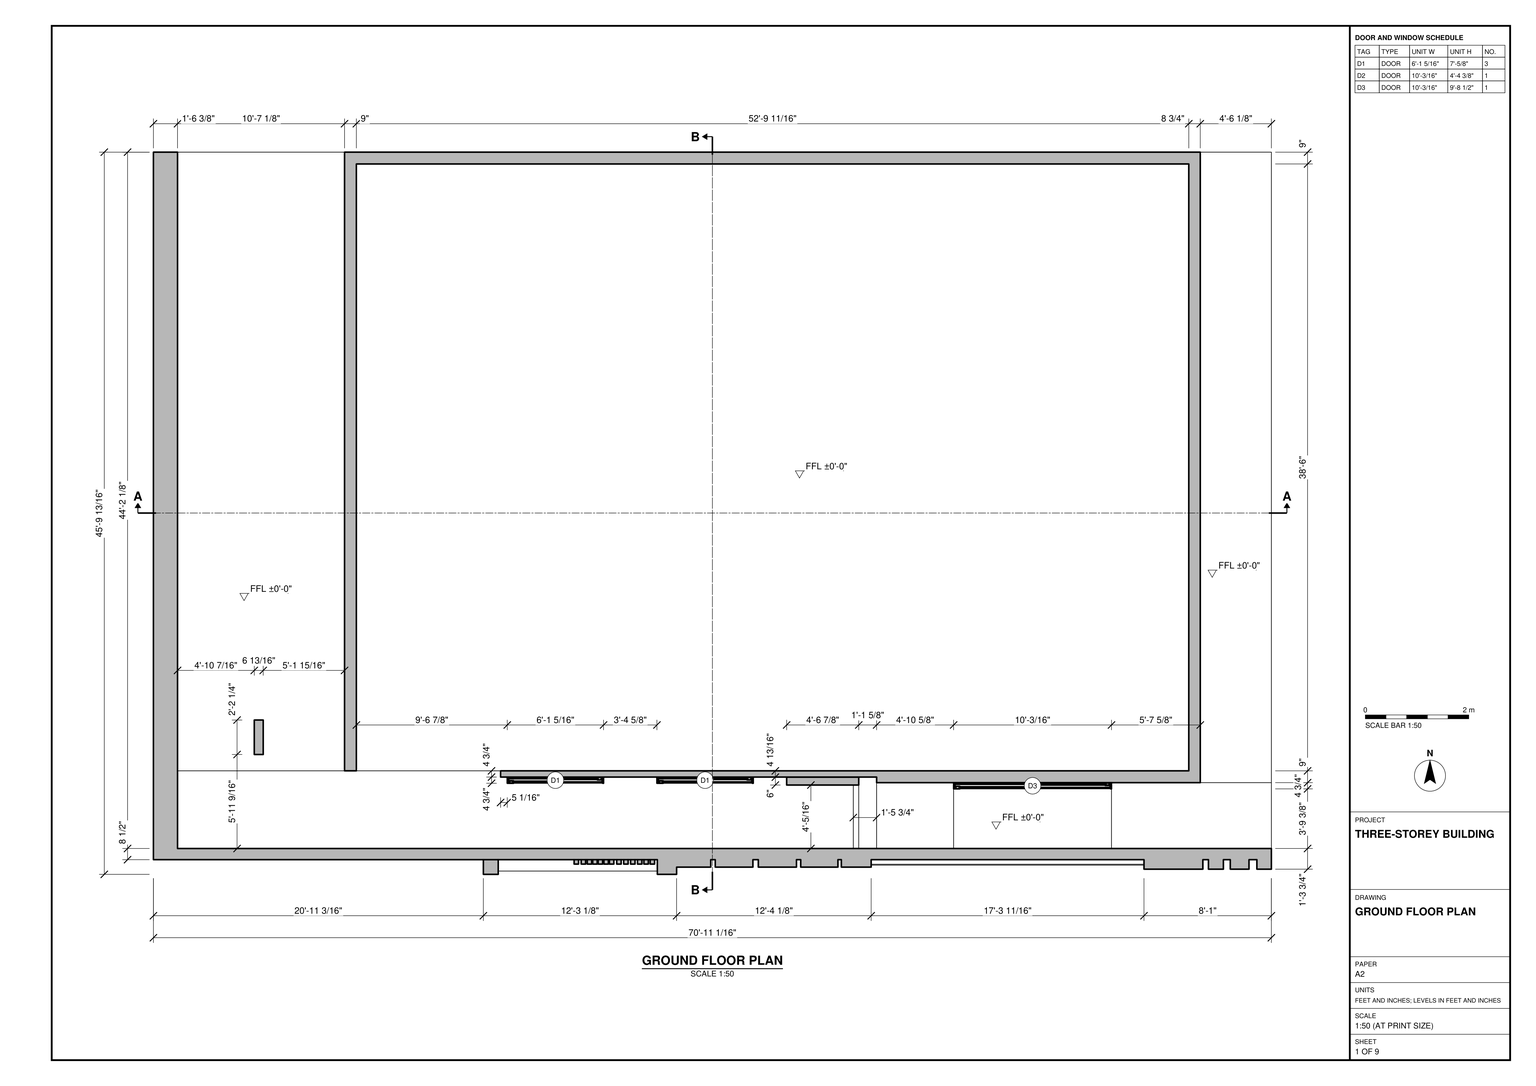
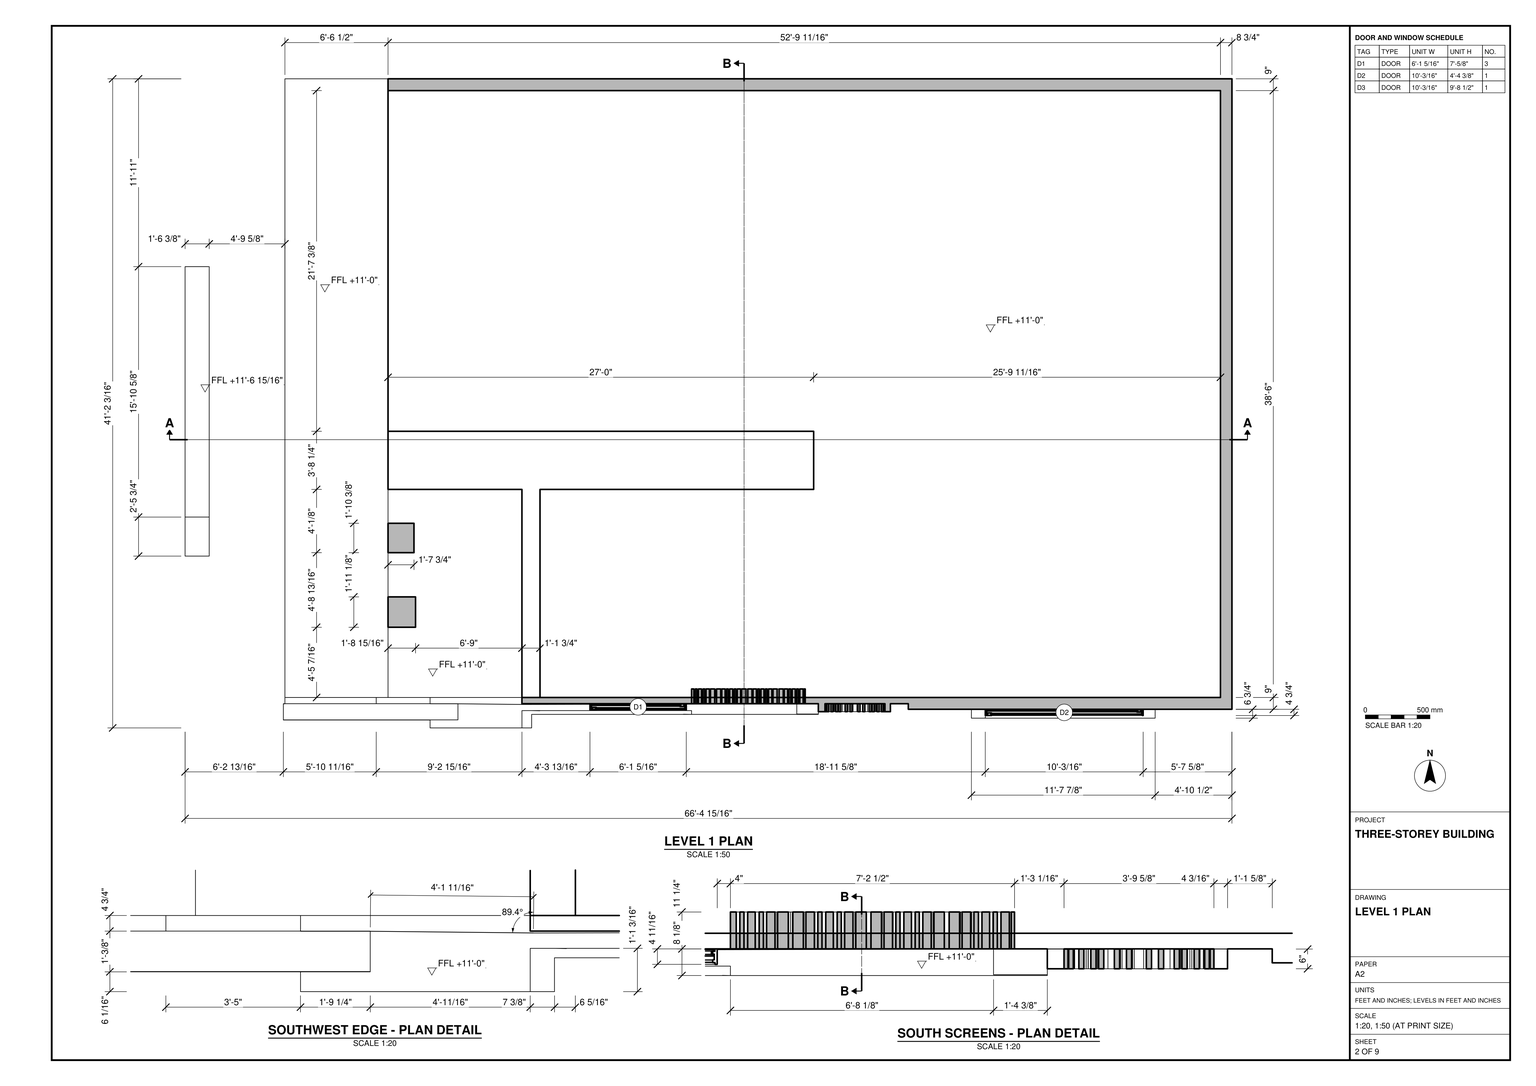
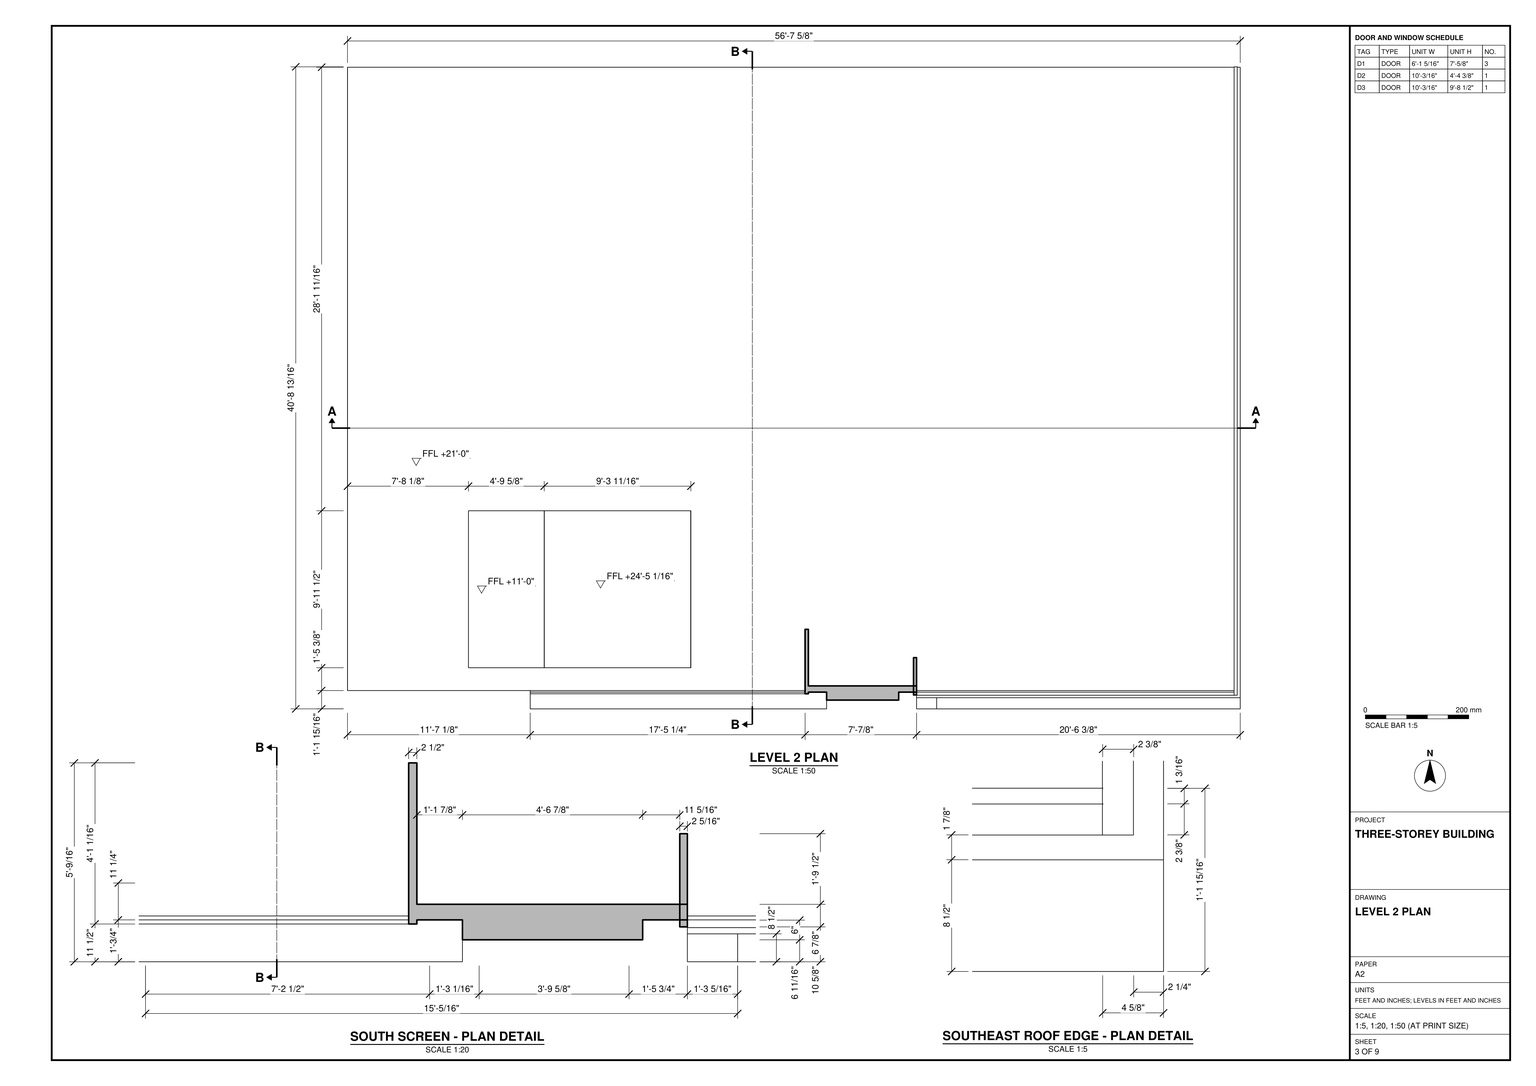
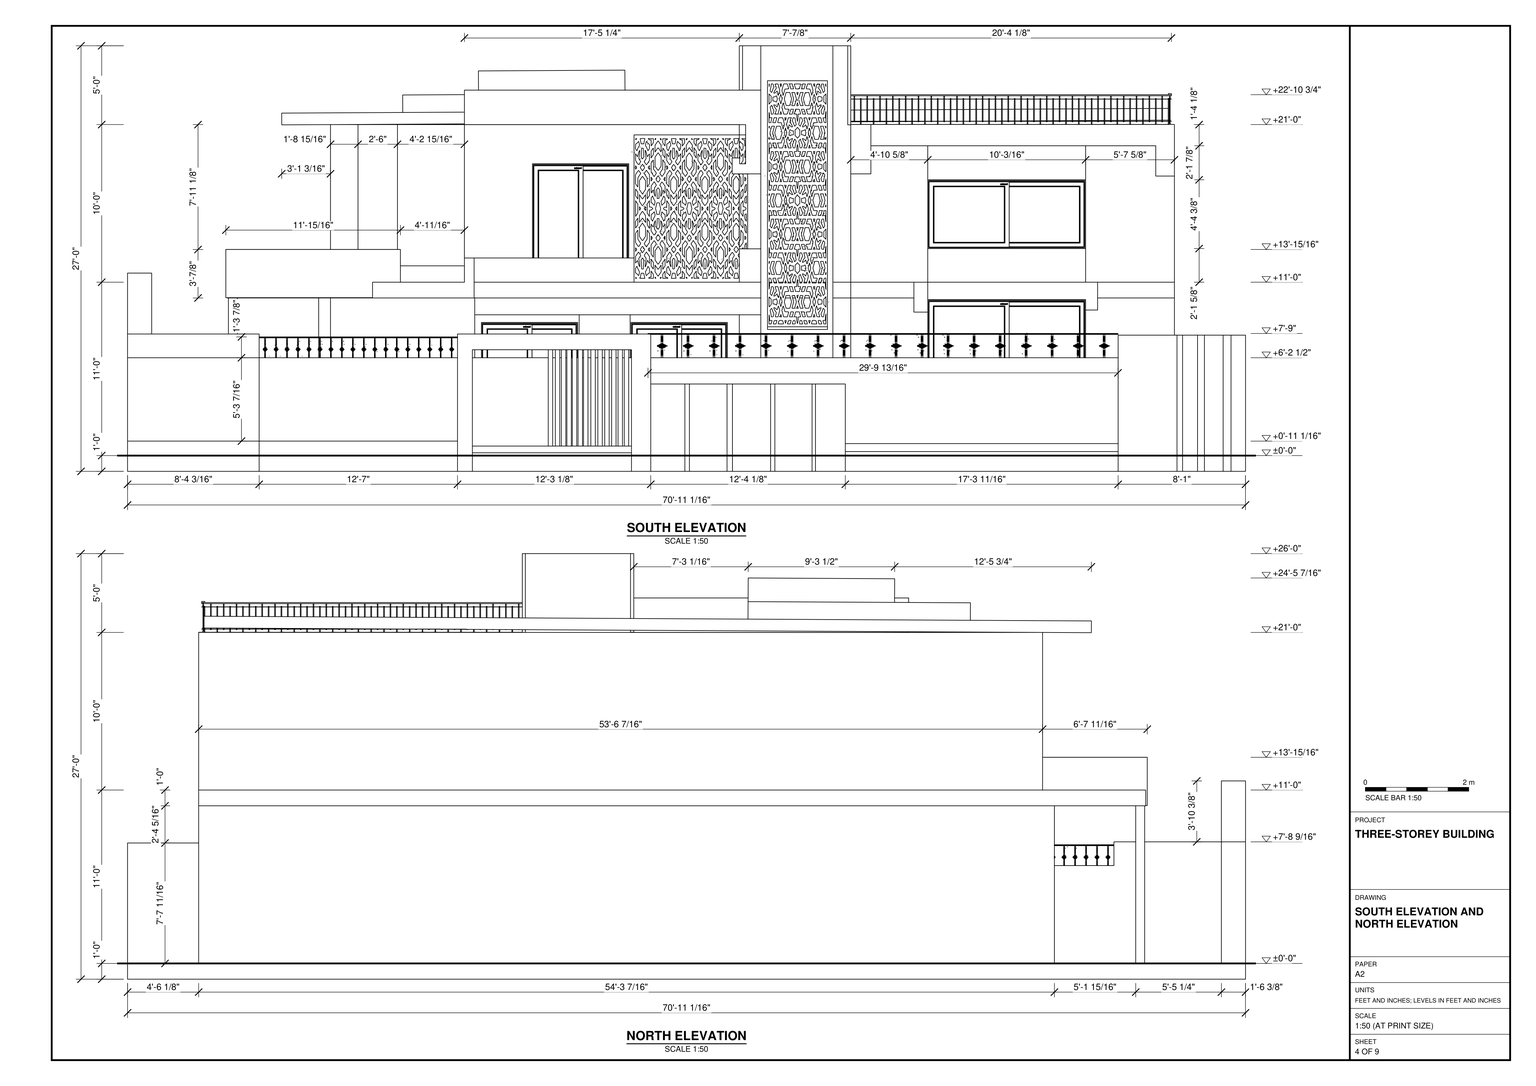
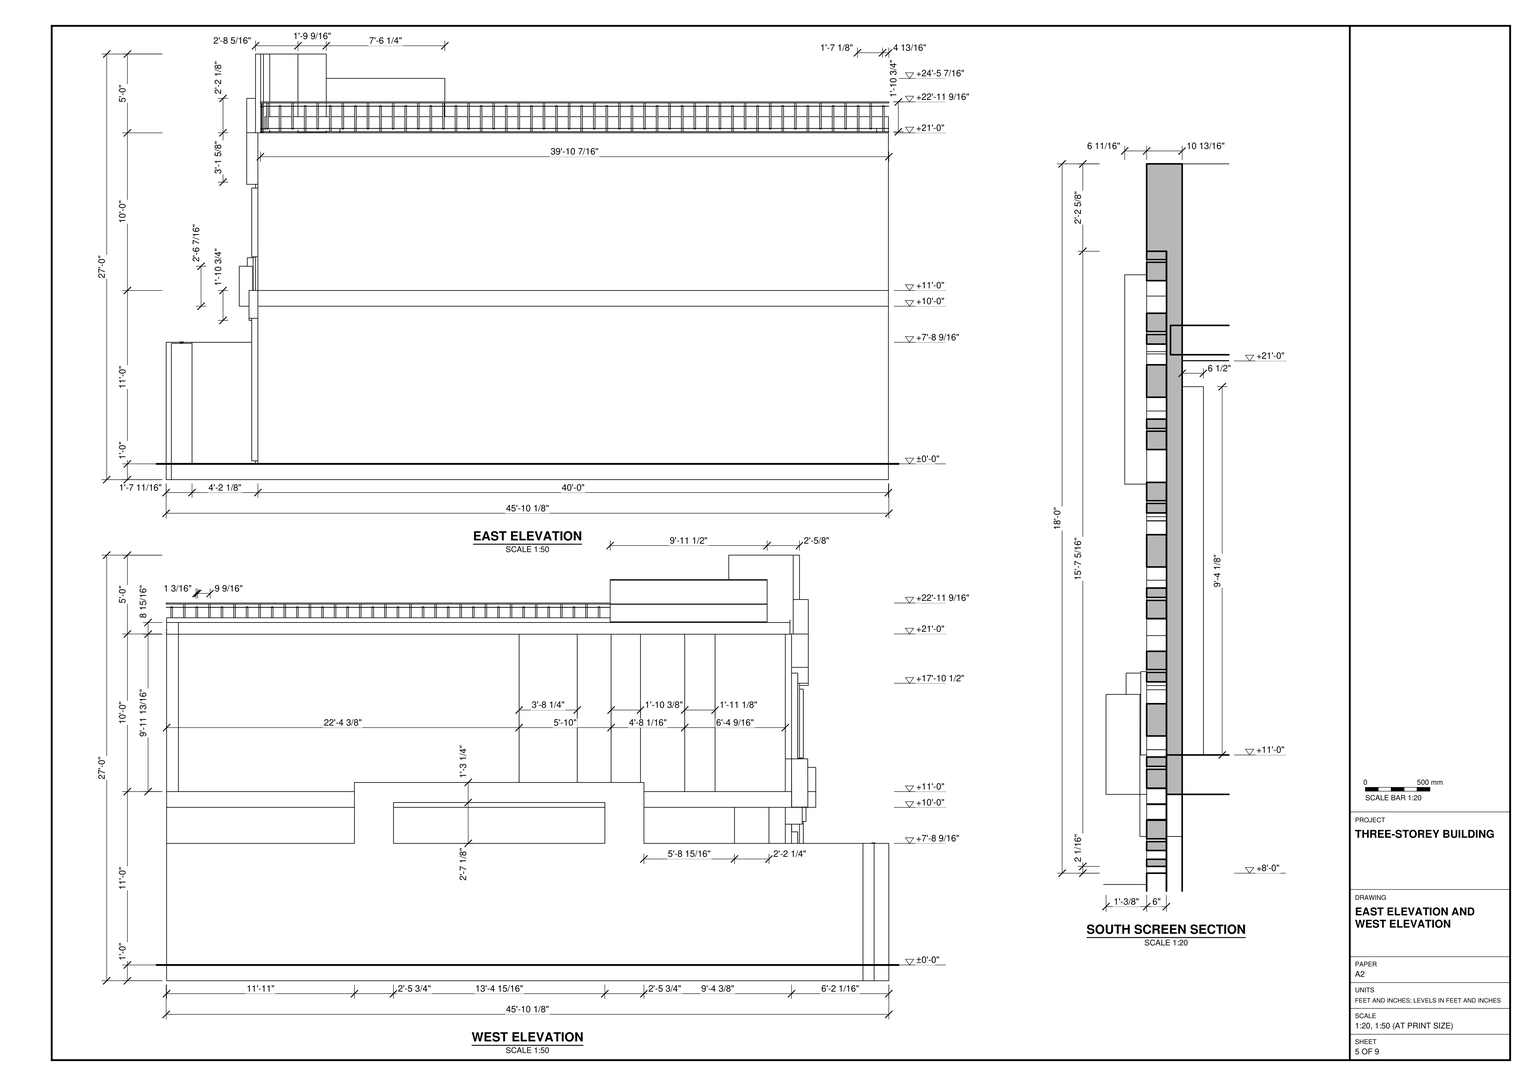
Build the three-storey building in SketchUp from task_files/diagram_01.pdf. Work in feet and inches. The overall model is 70'-11 1/16" wide from west to east, 45'-10 1/8" deep from south to north and 27'-0" high. Set the ground floor at ±0'-0", level 1 at +11'-0" and level 2 at +21'-0".

Lay out the main rectangular shell and the outer walls along its west and south sides. Keep the wider space beside the west wall and the narrower strip in front of the south facade. Use the wall thicknesses and offsets shown in plan. Place the framed sliding units according to the plans and opening schedule, distinguishing the fixed and sliding leaves. Model the floor slabs, the stepped southwest slab edge at level 1 and the two offset runs of south-facing screens. At roof level, retain the change in height within the southwest rectangular area and follow the enlarged details where the roof edge turns the southeast corner and meets the south screen.

Keep shell elements such as walls, slabs and roof, and any furniture or joinery pieces shown, in separate groups or components. Use components for repeated parts. Any decor or loose items shown may be suitable library components. Save one SketchUp model as output_files/three_storey_building_with_a_screened_south_elevation.skp.

# SketchUp Ruby script. Lengths in inches.
U = 1.inch
M = Sketchup.active_model
def pt(a) = Geom::Point3d.new(a.map { |v| v * U })
def face(e, loops, mat)
  f = e.add_face(loops[0].map { |a| pt(a) })
  loops[1..].each { |l| e.add_face(l.map { |a| pt(a) }).erase! }
  f.material = f.back_material = mat if mat
  f
end
# faces: each face lists its corners as indices into pts; further lists are holes
def faces(e, pts, list, mat = nil) = list.each { |f| face(e, (f[0].is_a?(Array) ? f : [f]).map { |l| l.map { |i| pts[i] } }, mat) }
# xy, xz, yz: faces in a plane at the given z, y or x. An outline is a flat list of corners, or four numbers for a rectangle; further outlines are holes
def ring(l) = l.size == 4 ? [[l[0], l[1]], [l[2], l[1]], [l[2], l[3]], [l[0], l[3]]] : l.each_slice(2).to_a
def flat(e, list, mat, &to3) = list.each { |f| face(e, (f[0].is_a?(Array) ? f : [f]).map { |l| ring(l).map { |u, v| to3.(u, v) } }, mat) }
def xy(e, z, list, mat = nil) = flat(e, list, mat) { |x, y| [x, y, z] }
def xz(e, y, list, mat = nil) = flat(e, list, mat) { |x, z| [x, y, z] }
def yz(e, x, list, mat = nil) = flat(e, list, mat) { |y, z| [x, y, z] }
def lines(e, pts, list) = list.each { |a, b| e.add_line(pt(pts[a]), pt(pts[b])) }
# prism: a flat outline (further loops are holes) pulled along v
def prism(e, loops, v, mat = nil)
  f = face(e, loops, mat); d = Geom::Vector3d.new(v.map { |x| x * U })
  f.pushpull(f.normal.samedirection?(d) ? d.length : -d.length)
end
def box(e, o, s, mat = nil) = prism(e, [[o, [o[0] + s[0], o[1], o[2]], [o[0] + s[0], o[1] + s[1], o[2]], [o[0], o[1] + s[1], o[2]]]], [0, 0, s[2]], mat)
def at(x, y, z, deg = 0) = Geom::Transformation.translation(pt([x, y, z])) * Geom::Transformation.rotation(ORIGIN, Z_AXIS, deg.degrees)
def axes(o, x, y, z) = Geom::Transformation.new([*x, 0, *y, 0, *z, 0, *pt(o).to_a, 1])
def part(name) = M.definitions.add(name)
# library, detail: a bought-in or finely detailed component or shape, given as its bounding box
def library(name, o, s) = part(name).tap { |d| box(d.entities, o, s) }
def detail(e, o, s) = box(e.add_group.entities, o, s)
def put(e, d, t, mat = nil) = e.add_instance(d, t).tap { |i| i.material = mat if mat }
def group(e, t, mat = nil) = e.add_group.tap { |g| g.transformation = t; g.material = mat if mat }.entities
root = M.entities
M.materials.add("[0119_RosyBrown]").color = [188, 143, 143]
M.materials.add("[Basic Tile]").color = [203, 206, 202]
M.materials.add("[Color G07]").color = [0, 153, 0]
M.materials.add("[Color M05]").color = [114, 114, 114]
M.materials.add("[Color M09]").color = [0, 0, 0]
M.materials.add("[Color_C21]").color = [51, 25, 0]
M.materials.add("[Slate Light Tile]").color = [54, 54, 54]
M.materials.add("[Translucent Glass Blue]").color = [100, 149, 237]
M.materials["[Translucent Glass Blue]"].alpha = 0.5
M.materials.add("[Wood Cherry Original]").color = [152, 86, 42]
M.materials.add("[Wood Floor Light]").color = [204, 176, 127]
M.materials.add("[Wood Veneer 02]").color = [190, 128, 91]
M.materials.add("[Wood_Floor_Parquet]").color = [145, 89, 39]
c1 = library("AS-120-mm",[0,0,0],[120.17,4.72,116.5])
c2 = library("AS-120-mm\#1",[0,0,0],[120.17,4.72,52.37])
c3 = library("GRC",[0,0,0],[45.06,0.39,22.46])
c4 = part("Group\#38")
xy(c4.entities,-1.02,[[0,0.34,0.39,0.73]])
xy(c4.entities,36.77,[[0,0.34,0.39,0.73]])
xz(c4.entities,0.34,[[0,-1.02,0.39,36.77]])
xz(c4.entities,0.73,[[0,-1.02,0.39,36.77]])
yz(c4.entities,0,[[0.34,-1.02,0.73,36.77]])
yz(c4.entities,0.39,[[0.34,-1.02,0.73,36.77]])
c5 = part("Raiing")
put(c5.entities,c4,at(0.98,124.07,1.02),"[Color_C21]")
put(c5.entities,c4,at(0.98,83.125,4.96),"[Color_C21]")
put(c5.entities,c4,at(0.98,1.23,4.96),"[Color_C21]")
put(c5.entities,c4,at(0.98,114.62,4.96),"[Color_C21]")
put(c5.entities,c4,at(0.98,133.52,4.96),"[Color_C21]")
put(c5.entities,c4,at(0.98,102.02,4.96),"[Color_C21]")
put(c5.entities,c4,at(0.98,35.88,1.02),"[Color_C21]")
put(c5.entities,c4,at(0.98,70.52,4.96),"[Color_C21]")
put(c5.entities,c4,at(0.98,130.37,1.02),"[Color_C21]")
put(c5.entities,c4,at(0.98,139.82,4.96),"[Color_C21]")
put(c5.entities,c4,at(0.98,26.43,4.96),"[Color_C21]")
put(c5.entities,c4,at(0.98,42.18,1.02),"[Color_C21]")
put(c5.entities,c4,at(0.98,146.12,4.96),"[Color_C21]")
put(c5.entities,c4,at(0.98,23.28,1.02),"[Color_C21]")
put(c5.entities,c4,at(0.98,95.72,4.96),"[Color_C21]")
put(c5.entities,c4,at(0.98,155.5625,1.02),"[Color_C21]")
put(c5.entities,c4,at(0.98,13.83,4.96),"[Color_C21]")
put(c5.entities,c4,at(0.98,86.27,1.02),"[Color_C21]")
put(c5.entities,c4,at(0.98,152.41,4.96),"[Color_C21]")
put(c5.entities,c4,at(0.98,108.32,4.96),"[Color_C21]")
put(c5.entities,c4,at(0.98,111.47,1.02),"[Color_C21]")
put(c5.entities,c4,at(0.98,142.97,1.02),"[Color_C21]")
put(c5.entities,c4,at(0.98,20.13,4.96),"[Color_C21]")
put(c5.entities,c4,at(0.98,92.57,1.02),"[Color_C21]")
put(c5.entities,c4,at(0.98,57.93,4.96),"[Color_C21]")
put(c5.entities,c4,at(0.98,51.63,4.96),"[Color_C21]")
put(c5.entities,c4,at(0.98,79.97,1.02),"[Color_C21]")
put(c5.entities,c4,at(0.98,61.08,1.02),"[Color_C21]")
put(c5.entities,c4,at(0.98,136.67,1.02),"[Color_C21]")
put(c5.entities,c4,at(0.98,105.17,1.02),"[Color_C21]")
put(c5.entities,c4,at(0.98,73.67,1.02),"[Color_C21]")
put(c5.entities,c4,at(0.98,98.87,1.02),"[Color_C21]")
put(c5.entities,c4,at(0.98,149.27,1.02),"[Color_C21]")
put(c5.entities,c4,at(0.98,45.33,4.96),"[Color_C21]")
put(c5.entities,c4,at(0.98,76.82,4.96),"[Color_C21]")
put(c5.entities,c4,at(0.98,64.23,4.96),"[Color_C21]")
put(c5.entities,c4,at(0.98,39.03,4.96),"[Color_C21]")
g1 = group(c5.entities,at(0,110.39,41.73),"[Wood_Floor_Parquet]")
box(g1,[0,-110.39,0],[2.36,157.49,1.57])
put(c5.entities,c4,at(0.98,16.98,1.02),"[Color_C21]")
put(c5.entities,c4,at(0.98,127.22,4.96),"[Color_C21]")
put(c5.entities,c4,at(0.98,117.77,1.02),"[Color_C21]")
put(c5.entities,c4,at(0.98,48.48,1.02),"[Color_C21]")
put(c5.entities,c4,at(0.98,67.375,1.02),"[Color_C21]")
put(c5.entities,c4,at(0.98,32.73,4.96),"[Color_C21]")
put(c5.entities,c4,at(0.98,10.68,1.02),"[Color_C21]")
put(c5.entities,c4,at(0.98,4.38,1.02),"[Color_C21]")
g2 = group(c5.entities,at(0.59,114.85,0),"[Color_C21]")
xy(g2,0,[[0,-114.85,0.79,42.625],[0.79,-114.85,1.18,42.625]])
xy(g2,0.16,[[0,-114.85,1.18,42.625]])
xz(g2,-114.85,[[0,0,1.18,0.16]])
xz(g2,42.625,[[0,0,1.18,0.16]])
yz(g2,0,[[-114.85,0,42.625,0.16]])
yz(g2,1.18,[[-114.85,0,42.625,0.16]])
put(c5.entities,c4,at(0.98,7.53,4.96),"[Color_C21]")
g3 = group(c5.entities,at(0.59,114.85,4.72),"[Color_C21]")
xy(g3,0,[[0,-114.85,1.18,42.625]])
xy(g3,0.16,[[0,-114.85,1.18,42.625]])
xz(g3,-114.85,[[0,0,1.18,0.16]])
xz(g3,42.625,[[0,0,1.18,0.16]])
yz(g3,0,[[-114.85,0,42.625,0.16]])
yz(g3,1.18,[[-114.85,0,42.625,0.16]])
put(c5.entities,c4,at(0.98,54.78,1.02),"[Color_C21]")
put(c5.entities,c4,at(0.98,120.92,4.96),"[Color_C21]")
put(c5.entities,c4,at(0.98,29.58,1.02),"[Color_C21]")
g4 = group(c5.entities,at(0.59,114.85,36.85),"[Color_C21]")
xy(g4,0,[[0,-114.85,0.79,42.625],[0.79,-114.85,1.18,42.625]])
xy(g4,0.16,[[0,-114.85,1.18,42.625]])
xz(g4,-114.85,[[0,0,1.18,0.16]])
xz(g4,42.625,[[0,0,1.18,0.16]])
yz(g4,0,[[-114.85,0,42.625,0.16]])
yz(g4,1.18,[[-114.85,0,42.625,0.16]])
put(c5.entities,c4,at(0.98,89.42,4.96),"[Color_C21]")
c6 = library("GRC\#1",[0,0,0],[45.06,0.39,22.46])
c7 = library("AS-120-mm\#2",[0,0,0],[73.3,4.72,84.62])
c8 = library("Box38",[151.65,-2.06,-0.13],[1.46,1.46,69.71])
c9 = part("Cylinder01")
p = [[-163.3125,-2.13,68.375],[-163.31,-2.55,68.68],[-163.31,-2.83,69.1],[-163.31,-2.93,69.57],[-163.31,-2.83,70.05],[-163.31,-2.55,70.47],
  [-163.31,-2.13,70.77],[-163.31,-1.61,70.9375],[-163.31,-1.05,70.9375],[-163.31,-0.53,70.77],[-163.31,-0.1,70.47],[-163.31,0.18,70.05],
  [-163.31,0.27,69.57],[-163.31,0.18,69.1],[-163.31,-0.1,68.68],[-163.3125,-0.53,68.375],[-163.3125,-1.05,68.21],[-163.3125,-1.61,68.21],
  [161.96,-2.93,69.55],[161.96,-2.83,69.08],[161.97,-2.55,68.66],[161.97,-2.13,68.35],[161.97,-1.61,68.1875],[161.97,-1.05,68.1875],
  [161.97,-0.53,68.35],[161.97,-0.1,68.66],[161.97,0.18,69.08],[161.96,0.27,69.55],[161.96,0.18,70.03],[161.96,-0.1,70.44],
  [161.96,-0.53,70.75],[161.96,-1.05,70.92],[161.96,-1.61,70.92],[161.96,-2.13,70.75],[161.96,-2.55,70.44],[161.96,-2.83,70.03]]
faces(c9.entities,p,[[0,1,2,3,4,5,6,7,8,9,10,11,12,13,14,15,16,17],[18,19,20,21,22,23,24,25,26,27,28,29,30,31,32,33,34,35],[17,22,21,0],[16,23,22,17],[15,24,23,16],[0,21,20,1],[14,25,24,15],[1,20,19,2],
  [13,26,25,14],[2,19,18,3],[12,27,26,13],[3,18,35,4],[11,28,27,12],[4,35,34,5],[10,29,28,11],[5,34,33,6],
  [9,30,29,10],[6,33,32,7],[8,31,30,9],[7,32,31,8]])
c10 = library("Loft01",[150.2,-4.32,27.54],[5.87,5.98,14.02])
c11 = library("Loft02",[149.13,-4.83,27.54],[5.98,5.97,14.02])
c12 = library("Loft03",[149.15,-3.78,27.54],[5.97,5.99,14.02])
c13 = part("skp235")
put(c13.entities,c8,at(0,0,0))
put(c13.entities,c9,at(0,0,0))
put(c13.entities,c10,at(0,0,0))
put(c13.entities,c11,at(0,0,0))
put(c13.entities,c12,at(0,0,0))
put(c13.entities,c11,at(-18,0,0))
put(c13.entities,c12,at(-18,0,0))
put(c13.entities,c8,at(-18,0,0))
put(c13.entities,c10,at(-18,0,0))
put(c13.entities,c10,at(-36,0,0))
put(c13.entities,c8,at(-36,0,0))
put(c13.entities,c12,at(-36,0,0))
put(c13.entities,c11,at(-36,0,0))
put(c13.entities,c11,at(-54,0,0))
put(c13.entities,c8,at(-54,0,0))
put(c13.entities,c10,at(-54,0,0))
put(c13.entities,c12,at(-54,0,0))
put(c13.entities,c12,at(-72,0,0))
put(c13.entities,c10,at(-72,0,0))
put(c13.entities,c8,at(-72,0,0))
put(c13.entities,c11,at(-72,0,0))
put(c13.entities,c12,at(-90,0,0))
put(c13.entities,c8,at(-90,0,0))
put(c13.entities,c10,at(-90,0,0))
put(c13.entities,c11,at(-90,0,0))
put(c13.entities,c11,at(-108,0,0))
put(c13.entities,c12,at(-108,0,0))
put(c13.entities,c8,at(-108,0,0))
put(c13.entities,c10,at(-108,0,0))
put(c13.entities,c10,at(-126,0,0))
put(c13.entities,c12,at(-126,0,0))
put(c13.entities,c8,at(-126,0,0))
put(c13.entities,c11,at(-126,0,0))
put(c13.entities,c12,at(-144,0,0))
put(c13.entities,c8,at(-144,0,0))
put(c13.entities,c10,at(-144,0,0))
put(c13.entities,c11,at(-144,0,0))
put(c13.entities,c10,at(-162,0,0))
put(c13.entities,c11,at(-162,0,0))
put(c13.entities,c12,at(-162,0,0))
put(c13.entities,c8,at(-162,0,0))
put(c13.entities,c10,at(-180,0,0))
put(c13.entities,c8,at(-180,0,0))
put(c13.entities,c11,at(-180,0,0))
put(c13.entities,c12,at(-180,0,0))
put(c13.entities,c11,at(-198,0,0))
put(c13.entities,c10,at(-198,0,0))
put(c13.entities,c8,at(-198,0,0))
put(c13.entities,c12,at(-198,0,0))
put(c13.entities,c8,at(-216,0,0))
put(c13.entities,c12,at(-216,0,0))
put(c13.entities,c10,at(-216,0,0))
put(c13.entities,c11,at(-216,0,0))
put(c13.entities,c8,at(-234,0,0))
put(c13.entities,c11,at(-234,0,0))
put(c13.entities,c10,at(-234,0,0))
put(c13.entities,c12,at(-234,0,0))
put(c13.entities,c11,at(-252,0,0))
put(c13.entities,c8,at(-252,0,0))
put(c13.entities,c10,at(-252,0,0))
put(c13.entities,c12,at(-252,0,0))
put(c13.entities,c11,at(-270,0,0))
put(c13.entities,c12,at(-270,0,0))
put(c13.entities,c8,at(-270,0,0))
put(c13.entities,c10,at(-270,0,0))
put(c13.entities,c8,at(-288,0,0))
put(c13.entities,c10,at(-288,0,0))
put(c13.entities,c12,at(-288,0,0))
put(c13.entities,c11,at(-288,0,0))
put(c13.entities,c11,at(-306,0,0))
put(c13.entities,c12,at(-306,0,0))
put(c13.entities,c10,at(-306,0,0))
put(c13.entities,c8,at(-306,0,0))
c14 = part("Railing1")
put(c14.entities,c13,at(154.11,1.88,0.13))
c15 = part("Group\#4")
box(c15.entities,[0,0,0],[3.375,92.8125,3.375])
xy(root,-12,[[[383.614,0,383.614,11.1875,0,11.1875,0,549.8125,851.0625,549.8125,851.0625,3.9375,840.021,3.9375,840.021,11.1875,834.027,11.1875,834.027,3.9375,819.769,3.9375,819.769,11.1875,814.533,11.1875,814.533,3.9375,803.142,3.9375,803.142,11.1875,798.907,11.1875,798.907,3.9375,754.09,3.9375,754.09,7,546.402,7,546.402,5.5,523.6875,5.5,523.6875,11.1875,521.101,11.1875,521.101,5.5,492.774,5.5,492.774,11.1875,489.537,11.1875,489.537,5.5,460.481,5.5,460.481,11.1875,456.374,11.1875,456.374,5.5,427.703,5.5,427.703,11.1875,424.261,11.1875,424.261,5.5,398.293,5.5,398.293,0],[154.5,78.8125,788.1875,540.8125]],[251.177,0,262.494,11.1875],[262.494,2.5,383.614,11.1875],[154.5,78.8125,788.1875,540.8125]],"[Basic Tile]")
xy(root,0,[[18.372,19.6875,532.792,19.6875,532.792,74,536.9375,74,536.9375,19.6875,550.551,19.6875,550.551,74.0625,264.288,74.0625,264.288,78.8125,18.372,78.8125],[532.792,19.6875,536.9375,68],[550.551,19.6875,609.166,69.8125],[609.166,19.6875,729.338,69.8125],[729.338,19.6875,851.0625,69.8125],
  [532.792,68,536.9375,74],[550.551,69.8125,796.9375,69.8125,796.9375,549.8125,145.5,549.8125,145.5,78.8125,154.5,78.8125,154.5,540.8125,788.1875,540.8125,788.1875,78.8125,264.288,78.8125,264.288,74.0625,550.551,74.0625],[796.9375,69.8125,851.0625,549.8125],[[18.372,78.8125,145.5,549.8125],[76.781,91.243,83.593,117.493]],[154.5,78.8125,788.1875,540.8125]],"[Basic Tile]")
xy(root,0.063,[[487.149,68,532.792,74]],"[Basic Tile]")
xy(root,0.4375,[[482.0625,68,487.149,74]],"[0119_RosyBrown]")
xy(root,2.125,[[262.494,2.5,383.614,11.1875]],"[Basic Tile]")
xy(root,3.0625,[[546.402,7,754.09,7.6875]],"[Basic Tile]")
xy(root,7.25,[[262.494,2.5,383.614,11.1875]],"[Color G07]")
xy(root,9.125,[[546.402,7.6875,754.09,11.1875]],"[Color G07]")
xy(root,54.509,[[398.293,5.5,424.261,11.1875],[427.703,5.5,456.374,11.1875],[460.481,5.5,489.537,11.1875],[492.774,5.5,521.101,11.1875],[523.6875,5.5,546.402,11.1875]],"[Basic Tile]")
xy(root,74.5,[[100.177,11.1875,754.09,19.6875]],"[Basic Tile]")
xy(root,80.594,[[262.494,0,383.614,11.1875]],"[Basic Tile]")
xy(root,91.6875,[[754.09,3.9375,798.907,3.9375,798.907,11.1875,803.142,11.1875,803.142,3.9375,814.533,3.9375,814.533,11.1875,819.769,11.1875,819.769,3.9375,834.027,3.9375,834.027,11.1875,840.021,11.1875,840.021,3.9375,851.0625,3.9375,851.0625,19.6875,754.09,19.6875]],"[Basic Tile]")
xy(root,92.5625,[[251.177,0,398.293,11.1875],[0,11.1875,100.177,19.6875],[0,19.6875,18.372,78.8125],[0,78.8125,18.372,186.435],[0,216.161,18.372,377.076],
  [0,406.802,18.372,549.8125]],"[Basic Tile]")
xy(root,96.001,[[487.149,68,532.792,74]],"[Basic Tile]")
xy(root,107.1875,[[264.288,65.9375,482.0625,74.0625]],"[Basic Tile]")
xy(root,110.8125,[[729.338,63.0625,738.463,69.8125]],"[Basic Tile]")
xy(root,118.774,[[609.166,63.0625,729.338,69.8125]],"[Basic Tile]")
xy(root,120,[[186.496,55.625,186.496,78.8125,264.288,78.8125,264.288,65.9375,263.822,65.9375,263.822,55.625],[264.288,65.9375,264.288,78.8125,788.1875,78.8125,788.1875,540.8125,154.5,540.8125,154.5,78.8125,145.5,78.8125,145.5,549.8125,796.9375,549.8125,796.9375,69.8125,550.551,69.8125,550.551,74.0625,482.0625,74.0625,482.0625,65.9375],[482.0625,74,550.551,74.0625],[76,74.0625,186.496,78.8125],[[76,78.8125,145.5,549.8125],[76.781,91.243,83.593,117.493]],
  [154.5,78.8125,788.1875,540.8125]],"[Basic Tile]")
xy(root,123.678,[[0,216.161,18.372,377.076]],"[Basic Tile]")
xy(root,132,[[186.496,55.625,256.434,55.625,256.434,68.8125,385.565,68.8125,385.565,65.9375,482.0625,65.9375,482.0625,74,465.684,74,257.403,73.48,207.72,74,186.496,74],[609.166,63.0625,738.463,69.8125],[385.565,65.9375,385.565,68.8125,264.222,68.8125],[550.551,69.8125,796.9375,69.8125,796.9375,549.8125,154.5,549.8125,154.5,540.8125,788.1875,540.8125,788.1875,78.8125,256.434,78.8125,256.434,74.0625,550.551,74.0625],[257.403,73.48,465.684,74,482.0625,74,482.0625,74.0625,256.434,74.0625,256.434,78.8125,186.496,78.8125,186.496,74,207.72,74],
  [482.0625,74,487.149,74.0625],[487.149,74,532.792,74.0625],[532.792,74,536.9375,74.0625],[536.9375,74,550.551,74.0625],[76,74.0625,186.496,78.8125],
  [76,78.8125,154.5,549.8125],[154.5,78.8125,256.434,78.8125,256.434,237.202,154.5,237.202,154.5,211.422,174.25,211.422,174.25,189.047,154.5,189.047,154.5,155.39,175.4375,155.39,175.4375,132.265,154.5,132.265],[270.192,78.8125,788.1875,78.8125,788.1875,540.8125,154.5,540.8125,154.5,281.452,478.5,281.452,478.5,237.202,270.192,237.202]],"[Basic Tile]")
xy(root,138.9375,[[0,186.435,18.372,216.161],[0,216.161,18.372,406.802]],"[Basic Tile]")
xy(root,150.4375,[[256.434,55.625,263.822,55.625,263.822,65.9375,385.565,65.9375,385.565,68.8125,256.434,68.8125]],"[Basic Tile]")
xy(root,212.811,[[782.72,61.3125,796.9375,69.8125]],"[Basic Tile]")
xy(root,214.476,[[460.264,61.3125,482.0625,74.0625]],"[Basic Tile]")
xy(root,222.16,[[465.951,61.3125,470.514,74.0625]],"[Basic Tile]")
xy(root,226.598,[[460.264,61.3125,465.951,74.0625]],"[Basic Tile]")
xy(root,235.874,[[565.863,61.3125,782.72,69.8125]],"[Basic Tile]")
xy(root,251.9375,[[256.434,72.8125,465.684,74.0625],[465.684,72.8125,468.184,74.0625]],"[Basic Tile]")
xy(root,252,[[550.551,69.8125,796.9375,69.8125,796.9375,549.8125,154.5,549.8125,154.5,540.8125,788.1875,540.8125,788.1875,78.8125,550.551,78.8125],[256.434,74.0625,465.684,78.8125],[256.434,78.8125,270.192,237.202],[154.5,132.265,175.4375,155.39],[154.5,189.047,174.25,211.422],
  [154.5,237.202,478.5,281.452]],"[Basic Tile]")
xy(root,252.101,[[565.863,61.3125,796.9375,69.8125]],"[Basic Tile]")
xy(root,252.125,[[465.684,78.8125,468.184,121.875]],"[Basic Tile]")
xy(root,278.229,[[256.434,61.3125,482.0625,61.3125,482.0625,74.0625,468.184,74.0625,468.184,72.8125,256.434,72.8125]],"[Basic Tile]")
xy(root,285.388,[[487.149,68,532.792,74.0625]],"[0119_RosyBrown]")
xy(root,312,[[482.0625,68,536.9375,68,536.9375,74.0625,550.551,74.0625,550.551,78.8125,468.184,78.8125,468.184,74.0625,482.0625,74.0625],[465.684,72.8125,468.184,121.875]],"[Basic Tile]")
xz(root,0,[[251.177,-12,262.494,-12,262.494,80.594,383.614,80.594,383.614,-12,398.293,-12,398.293,92.5625,251.177,92.5625]],"[Basic Tile]")
xz(root,2.5,[[262.494,2.125,383.614,7.25]],"[Color G07]")
xz(root,2.5,[[262.494,-12,383.614,2.125]],"[Wood Veneer 02]")
xz(root,3.9375,[[754.09,-12,798.907,91.6875],[803.142,-12,814.533,91.6875],[819.769,-12,834.027,91.6875],[840.021,-12,851.0625,91.6875]],"[Wood Floor Light]")
xz(root,5.5,[[398.293,-12,424.261,54.509],[427.703,-12,456.374,54.509],[460.481,-12,489.537,54.509],[492.774,-12,521.101,54.509],[523.6875,-12,546.402,54.509]],"[Color M05]")
xz(root,7,[[546.402,-12,754.09,3.0625]],"[Wood Veneer 02]")
xz(root,7.6875,[[546.402,3.0625,754.09,9.125]],"[Color G07]")
xz(root,11.1875,[[251.177,-12,262.494,74.5],[262.494,-12,383.614,2.125],[424.261,-12,427.703,54.509],[456.374,-12,460.481,54.509],[489.537,-12,492.774,54.509],
  [521.101,-12,523.6875,54.509],[798.907,-12,803.142,91.6875],[814.533,-12,819.769,91.6875],[834.027,-12,840.021,91.6875],[262.494,2.125,383.614,7.25],
  [546.402,9.125,754.09,9.125,754.09,74.5,398.293,74.5,398.293,54.509,546.402,54.509],[100.177,11.036,251.177,74.5],[251.177,74.5,251.177,92.5625,398.293,92.5625,398.293,74.5,383.614,74.5,383.614,80.594,262.494,80.594,262.494,74.5]],"[Basic Tile]")
xz(root,11.1875,[[0,-12,100.177,11.036],[100.177,-12,251.177,11.036],[0,11.036,100.177,74.5],[0,74.5,100.177,92.5625]],"[Color M05]")
xz(root,11.1875,[[262.494,7.25,383.614,74.5]],"[Wood Floor Light]")
xz(root,19.6875,[[18.372,0,18.372,92.5625,100.177,92.5625,100.177,74.5,754.09,74.5,754.09,91.6875,851.0625,91.6875,851.0625,0]],"[Basic Tile]")
xz(root,55.625,[[186.496,120,263.822,120,263.822,150.4375,256.434,150.4375,256.434,132,186.496,132]],"[Basic Tile]")
xz(root,61.3125,[[782.72,212.811,796.9375,212.811,796.9375,252.101,565.863,252.101,565.863,235.874,782.72,235.874],[460.264,214.476,482.0625,214.476,482.0625,278.229,256.434,278.229,256.434,251.9375,470.514,251.9375,470.514,222.16,465.951,222.16,465.951,226.598,460.264,226.598]],"[Basic Tile]")
xz(root,63.0625,[[729.338,110.8125,738.463,110.8125,738.463,132,609.166,132,609.166,118.774,729.338,118.774]],"[Basic Tile]")
xz(root,65.9375,[[264.288,107.1875,482.0625,120],[263.822,120,482.0625,132],[263.822,132,385.565,150.4375]],"[Basic Tile]")
xz(root,68,[[[532.792,0,536.9375,0,536.9375,312,482.0625,312,482.0625,0.4375,487.149,0.4375,487.149,0.063,532.792,0.063],[487.149,96.001,532.792,285.388]]],"[Wood Floor Light]")
xz(root,68.8125,[[256.434,132,385.565,150.4375]],"[Basic Tile]")
xz(root,69.8125,[[609.166,0,729.338,118.774],[729.338,110.8125,738.463,120],[609.166,118.774,729.338,120],[609.166,120,738.463,132],[782.72,212.811,782.72,235.874,729.338,235.874,729.338,252,796.9375,252,796.9375,212.811],
  [565.863,235.874,609.166,252],[609.166,235.874,729.338,252],[565.863,252,796.9375,252.101]],"[Basic Tile]")
xz(root,69.8125,[[609.166,132,729.338,235.874]],"[Wood Cherry Original]")
xz(root,69.8125,[[550.551,0,609.166,120],[729.338,0,796.9375,0,796.9375,120,738.463,120,738.463,110.8125,729.338,110.8125],[550.551,120,609.166,132],[738.463,120,796.9375,132],[550.551,132,609.166,132,609.166,235.874,565.863,235.874,565.863,252,550.551,252],
  [729.338,132,796.9375,132,796.9375,212.811,782.72,212.811,782.72,235.874,729.338,235.874]],"[Wood Floor Light]")
xz(root,72.8125,[[256.434,251.9375,465.684,278.229],[465.684,251.9375,468.184,278.229],[465.684,278.229,468.184,312]],"[Basic Tile]")
xz(root,74,[[532.792,0,536.9375,120],[482.0625,0.4375,487.149,120]],"[0119_RosyBrown]")
xz(root,74,[[487.149,0.063,532.792,96.001],[487.149,96.001,532.792,120],[482.0625,120,487.149,132],[487.149,120,532.792,132],[532.792,120,536.9375,132],
  [536.9375,120,550.551,132]],"[Basic Tile]")
xz(root,74.0625,[[264.288,0,343.807,107.1875],[382.589,0,550.551,0,550.551,120,536.9375,120,536.9375,98.0625,482.0625,98.0625,482.0625,107.1875,382.589,107.1875],[482.0625,98.0625,487.149,120],[487.149,98.0625,532.792,120],[532.792,98.0625,536.9375,120],
  [76,120,186.496,132],[482.0625,120,487.149,132],[487.149,120,532.792,132],[532.792,120,536.9375,132],[487.149,132,532.792,285.388],
  [536.9375,132,550.551,132,550.551,284,549.613,284,549.613,312,536.9375,312],[468.184,278.229,482.0625,312],[549.613,298.0625,550.551,312]],"[Basic Tile]")
xz(root,74.0625,[[343.807,0,382.589,107.1875]],"[Wood Cherry Original]")
xz(root,74.0625,[[256.434,132,482.0625,132,482.0625,214.476,460.264,214.476,460.264,226.598,465.951,226.598,465.951,222.16,470.514,222.16,470.514,251.9375,256.434,251.9375],[256.434,251.9375,465.684,252]],"[Wood Floor Light]")
xz(root,75.265,[[117.376,251.803,117.328,260.74,792.826,264.33,792.874,255.392]],"[Basic Tile]")
xz(root,78.8125,[[154.5,-12,788.1875,0],[145.5,0,154.5,120],[264.288,0,788.1875,120],[154.5,120,788.1875,132],[256.434,132,270.192,252],
  [270.192,132,270.192,252,465.684,252,465.684,252.125,468.184,252.125,468.184,312,550.551,312,550.551,252,788.1875,252,788.1875,132]],"[Basic Tile]")
xz(root,91.243,[[76.781,0,83.593,120]],"[Color M05]")
xz(root,92.635,[[209.501,261.23,209.43,274.542,267.179,274.849,378.678,275.442,378.749,262.129]],"[Basic Tile]")
xz(root,92.635,[[267.179,274.849,378.678,275.442,378.582,293.441,267.084,292.849]],"[Slate Light Tile]")
xz(root,117.493,[[76.781,0,83.593,120]],"[Basic Tile]")
xz(root,121.875,[[465.684,252.125,468.184,312]],"[Basic Tile]")
xz(root,132.265,[[154.5,132,175.4375,252]],"[Basic Tile]")
xz(root,155.39,[[154.5,132,175.4375,252]],"[Basic Tile]")
xz(root,186.435,[[0,92.5625,18.372,138.9375]],"[Basic Tile]")
xz(root,189.047,[[154.5,132,174.25,252]],"[Basic Tile]")
xz(root,211.422,[[154.5,132,174.25,252]],"[Basic Tile]")
xz(root,212.135,[[209.501,261.23,378.749,262.129,378.678,275.442,267.179,274.849,209.43,274.542],[267.179,274.849,267.084,292.849,378.582,293.441,378.678,275.442]],"[Basic Tile]")
xz(root,216.161,[[0,92.5625,18.372,123.678]],"[Basic Tile]")
xz(root,237.202,[[205.467,132,256.434,252],[270.192,132,478.5,252]],"[Basic Tile]")
xz(root,237.202,[[154.5,132,205.467,252]],"[Wood Cherry Original]")
xz(root,281.452,[[154.5,132,478.5,252]],"[Basic Tile]")
xz(root,377.076,[[0,92.5625,18.372,123.678]],"[Basic Tile]")
xz(root,406.802,[[0,92.5625,18.372,138.9375]],"[Basic Tile]")
xz(root,540.8125,[[154.5,-12,788.1875,0],[154.5,0,788.1875,120],[154.5,120,788.1875,132],[154.5,132,788.1875,252]],"[Basic Tile]")
xz(root,549.8125,[[0,-12,0,92.5625,18.372,92.5625,18.372,0,851.0625,0,851.0625,-12],[145.5,0,796.9375,120],[76,120,796.9375,132],[154.5,132,796.9375,252],[117.376,251.803,154.5,252,792.874,255.392,792.826,264.33,117.328,260.74]],"[Basic Tile]")
yz(root,0,[[11.1875,-12,19.6875,92.5625],[[19.6875,-12,19.6875,92.5625,186.435,92.5625,186.435,138.9375,406.802,138.9375,406.802,92.5625,549.8125,92.5625,549.8125,-12],[216.161,92.5625,377.076,123.678]]],"[Basic Tile]")
yz(root,18.372,[[19.6875,0,78.8125,92.5625],[[78.8125,0,549.8125,0,549.8125,92.5625,406.802,92.5625,406.802,138.9375,186.435,138.9375,186.435,92.5625,78.8125,92.5625],[216.161,92.5625,377.076,123.678]]],"[Basic Tile]")
yz(root,74.8125,[[73.97,120.1875,61.658,120.218,61.75,156.942,74.0625,156.911]],"[Basic Tile]")
yz(root,76,[[74.0625,120,549.8125,132]],"[Basic Tile]")
yz(root,76.781,[[91.243,0,117.493,120]],"[Basic Tile]")
yz(root,83.593,[[91.243,0,117.493,120]],"[Color M05]")
yz(root,100.177,[[11.1875,74.5,19.6875,92.5625]],"[Basic Tile]")
yz(root,145.5,[[78.8125,0,549.8125,120]],"[Basic Tile]")
yz(root,154.5,[[78.8125,-12,540.8125,0],[78.8125,0,540.8125,120],[78.8125,120,540.8125,132],[132.265,132,155.39,252],[189.047,132,211.422,252],
  [237.202,132,281.452,252],[281.452,132,540.8125,252],[540.8125,132,549.8125,252]],"[Basic Tile]")
yz(root,174.25,[[189.047,132,211.422,252]],"[Basic Tile]")
yz(root,175.4375,[[132.265,132,155.39,252]],"[Basic Tile]")
yz(root,186.496,[[55.625,120,74.0625,132]],"[Basic Tile]")
yz(root,207.72,[[73.97,120.1875,74,132,74.031,144.456,74.0625,156.911,61.75,156.942,61.658,120.218]],"[Basic Tile]")
yz(root,251.177,[[0,-12,11.1875,92.5625]],"[Basic Tile]")
yz(root,256.434,[[55.625,132,68.8125,150.4375],[74.0625,132,78.8125,252],[78.8125,132,237.202,252],[61.3125,251.9375,72.8125,278.229]],"[Basic Tile]")
yz(root,262.494,[[0,-12,2.5,-12,2.5,7.25,11.1875,7.25,11.1875,80.594,0,80.594],[2.5,2.125,11.1875,7.25]],"[Basic Tile]")
yz(root,263.822,[[55.625,120,65.9375,150.4375]],"[Basic Tile]")
yz(root,264.288,[[74.0625,0,78.8125,107.1875],[65.9375,107.1875,78.8125,120]],"[Basic Tile]")
yz(root,270.192,[[78.8125,132,237.202,252]],"[Basic Tile]")
yz(root,383.614,[[0,-12,0,80.594,11.1875,80.594,11.1875,7.25,2.5,7.25,2.5,-12],[2.5,2.125,11.1875,7.25]],"[Basic Tile]")
yz(root,385.565,[[65.9375,132,68.8125,150.4375]],"[Basic Tile]")
yz(root,398.293,[[0,-12,5.5,-12,5.5,54.509,11.1875,54.509,11.1875,92.5625,0,92.5625]],"[Basic Tile]")
yz(root,424.261,[[5.5,-12,11.1875,54.509]],"[Basic Tile]")
yz(root,427.703,[[5.5,-12,11.1875,54.509]],"[Basic Tile]")
yz(root,456.374,[[5.5,-12,11.1875,54.509]],"[Basic Tile]")
yz(root,460.264,[[61.3125,214.476,74.0625,226.598]],"[Basic Tile]")
yz(root,460.481,[[5.5,-12,11.1875,54.509]],"[Basic Tile]")
yz(root,465.684,[[74,132,66.19,132.004,66.204,157.404,74.013,157.4],[72.8125,251.9375,72.8125,312,121.875,312,121.875,252.125,78.8125,252.125,78.8125,252,74.0625,252,74.0625,251.9375]],"[Basic Tile]")
yz(root,465.951,[[61.3125,222.16,74.0625,226.598]],"[Basic Tile]")
yz(root,468.184,[[72.8125,251.9375,74.0625,278.229],[78.8125,252.125,121.875,312],[72.8125,278.229,74.0625,312]],"[Basic Tile]")
yz(root,470.514,[[61.3125,222.16,74.0625,251.9375]],"[Basic Tile]")
yz(root,478.5,[[237.202,132,281.452,252]],"[Basic Tile]")
yz(root,482.0625,[[68,0.4375,74,107.1875],[68,107.1875,74,120],[68,120,74,132],[68,132,68,132.003,74,132],[74,132,68,132.003,68,157.404,74.013,157.4],
  [74,132,74.013,157.4,68,157.404,68,214.476,74.0625,214.476,74.0625,132],[68,278.229,74.0625,312]],"[0119_RosyBrown]")
yz(root,482.0625,[[65.9375,107.1875,68,120],[74,107.1875,74.0625,120],[65.9375,120,68,132],[68,132.003,68,157.404,66.204,157.404,66.19,132.004],[61.3125,214.476,68,278.229]],"[Basic Tile]")
yz(root,487.149,[[68,0.063,74,0.4375],[68,96.001,74,96.001,74,132,74.0625,132,74.0625,285.388,68,285.388]],"[0119_RosyBrown]")
yz(root,489.537,[[5.5,-12,11.1875,54.509]],"[Basic Tile]")
yz(root,492.774,[[5.5,-12,11.1875,54.509]],"[Basic Tile]")
yz(root,521.101,[[5.5,-12,11.1875,54.509]],"[Basic Tile]")
yz(root,523.6875,[[5.5,-12,11.1875,54.509]],"[Basic Tile]")
yz(root,532.792,[[68,0,74,0.063],[68,96.001,68,285.388,74.0625,285.388,74.0625,132,74,132,74,96.001]],"[0119_RosyBrown]")
yz(root,536.9375,[[68,0,74,0,74,132,74.0625,132,74.0625,312,68,312]],"[0119_RosyBrown]")
yz(root,546.402,[[5.5,-12,7,3.0625],[5.5,3.0625,7.6875,9.125],[5.5,9.125,11.1875,54.509]],"[Basic Tile]")
yz(root,550.551,[[69.8125,0,74.0625,120],[69.8125,120,74,132],[69.8125,132,74.0625,252],[74.0625,252,78.8125,312]],"[Basic Tile]")
yz(root,565.863,[[61.3125,235.874,69.8125,252.101]],"[Basic Tile]")
yz(root,609.166,[[63.0625,118.774,69.8125,132]],"[Basic Tile]")
yz(root,729.338,[[63.0625,110.8125,69.8125,118.774]],"[Basic Tile]")
yz(root,738.463,[[63.0625,110.8125,69.8125,132]],"[Basic Tile]")
yz(root,754.09,[[3.9375,-12,3.9375,91.6875,11.1875,91.6875,11.1875,9.125,7.6875,9.125,7.6875,3.0625,7,3.0625,7,-12],[11.1875,74.5,19.6875,91.6875]],"[Basic Tile]")
yz(root,782.72,[[61.3125,212.811,69.8125,235.874]],"[Basic Tile]")
yz(root,788.1875,[[78.8125,-12,540.8125,0],[78.8125,0,540.8125,120],[78.8125,120,540.8125,132],[78.8125,132,540.8125,252]],"[Basic Tile]")
yz(root,796.9375,[[69.8125,0,549.8125,120],[69.8125,120,549.8125,132],[69.8125,132,549.8125,252],[61.3125,212.811,69.8125,252.101]],"[Basic Tile]")
yz(root,798.907,[[3.9375,-12,11.1875,91.6875]],"[Basic Tile]")
yz(root,803.142,[[3.9375,-12,11.1875,91.6875]],"[Basic Tile]")
yz(root,814.533,[[3.9375,-12,11.1875,91.6875]],"[Basic Tile]")
yz(root,819.769,[[3.9375,-12,11.1875,91.6875]],"[Basic Tile]")
yz(root,834.027,[[3.9375,-12,11.1875,91.6875]],"[Basic Tile]")
yz(root,840.021,[[3.9375,-12,11.1875,91.6875]],"[Basic Tile]")
yz(root,851.0625,[[3.9375,-12,549.8125,0],[3.9375,0,19.6875,91.6875]],"[Basic Tile]")
p = [[207.72,61.658,120.218],[207.72,61.75,156.942],[74.8125,61.75,156.942],[74.8125,61.658,120.218],[186.496,73.97,120.1875],[207.72,73.97,120.1875],
  [74.8125,73.97,120.1875],[207.72,74.0625,156.911],[207.72,74.031,144.456],[207.72,74,132],[186.496,74,132],[74.8125,74.0625,156.911],
  [145.5,74.0625,156.911],[465.684,66.204,157.404],[465.684,66.19,132.004],[482.0625,66.19,132.004],[482.0625,66.204,157.404],[465.684,74,132],
  [482.0625,74,132],[482.0625,68,132.003],[257.403,73.511,144.456],[257.403,73.48,132],[465.684,74.013,157.4],[482.0625,74.013,157.4],
  [482.0625,68,157.404],[117.376,281.452,251.803],[117.376,540.8125,251.803],[117.328,540.8125,260.74],[117.328,75.265,260.74],[117.376,75.265,251.803],
  [117.376,132.265,251.803],[117.376,155.39,251.803],[117.376,189.047,251.803],[117.376,211.422,251.803],[117.376,237.202,251.803],[792.874,132.265,255.392],
  [154.5,132.265,252],[792.874,75.265,255.392],[154.5,155.39,252],[154.5,189.047,252],[154.5,211.422,252],[154.5,237.202,252],
  [154.5,281.452,252],[154.5,540.8125,252],[117.376,549.8125,251.803],[117.328,549.8125,260.74],[154.5,549.8125,252],[792.874,549.8125,255.392],
  [792.826,75.265,264.33],[792.826,549.8125,264.33],[209.501,92.635,261.23],[378.749,92.635,262.129],[378.749,212.135,262.129],[209.501,212.135,261.23],
  [209.43,212.135,274.542],[209.43,92.635,274.542],[378.678,92.635,275.442],[378.678,212.135,275.442],[267.179,212.135,274.849],[267.179,92.635,274.849],
  [267.084,92.635,292.849],[267.084,212.135,292.849],[378.582,212.135,293.441],[378.582,92.635,293.441],[465.684,74,120],[465.684,73.9375,0],
  [465.684,74.0625,251.9375],[145.5,78.8125,156.911]]
faces(root,p,[[0,1,2,3]],"[Wood Cherry Original]")
faces(root,p,[[4,5,0,3,6],[7,8,9,10,4,6,11,12],[10,9,5,4],[13,14,15,16],[17,18,19,15,14],[17,22,23,18],[7,12,11,2,1],[23,22,13,16,24],
  [25,26,27,28,29,30,31,32,33,34],[35,36,30,29,37],[36,38,31,30],[38,39,32,31],[39,40,33,32],[40,41,34,33],[41,42,25,34],[42,43,26,25],
  [26,44,45,27],[43,46,44,26],[47,35,37,48,49],[[28,27,45,49,48],[50,51,52,53]],[50,53,54,55],[52,51,56,57],[55,54,58,59],[58,59,60,61],
  [58,57,56,59],[56,57,62,63],[60,63,62,61]],"[Basic Tile]")
faces(root,p,[[20,21,9,8]],"[Translucent Glass Blue]")
lines(root,p,[[64,65],[22,66],[12,67]])
put(root,c1,at(609.17,65.09,2.26),"[Wood Cherry Original]")
put(root,c2,at(609.17,65.09,157.61),"[Basic Tile]")
put(root,c3,axes([487.15,68,285.39],[0,0,-4.1577],[0,15.24,0],[2.03177,0,0]),"[Basic Tile]")
put(root,c5,axes([550.55,74.0625,252],[0,-1,0],[1.55,0,0],[0,0,0.5254]),"[Basic Tile]")
put(root,c5,axes([792.28,71.7,252.83],[1,0,0],[0,3.038,0],[0,0,0.5254]),"[Basic Tile]")
put(root,c6,axes([385.56,74.0625,132],[1.92014,0,0],[0,28.51599,0],[0,0,4.9924]),"[Basic Tile]")
put(root,c7,at(308.24,69.34,137.58),"[Wood Cherry Original]")
put(root,c7,at(383.31,69.34,16.75),"[Wood Cherry Original]")
put(root,c7,at(269.37,69.34,16.75),"[Wood Cherry Original]")
put(root,c14,axes([406.3,11.1875,74.5],[1.1,0,0],[0,1,0],[0,0,0.26]),"[Basic Tile]")
put(root,c14,axes([104.45,13.3,71.87],[0.46422,0,0],[0,0.71568,0],[0,0,0.26]),"[Basic Tile]")
g5 = group(root,at(550.55,69.8125,214.48),"[Basic Tile]")
box(g5,[0,-8.5,0],[15.3125,8.5,37.625])
g6 = group(root,at(600.48,69.8125,106.1),"[Basic Tile]")
box(g6,[-1.875,-6.75,3.125],[10.5625,6.75,22.78])
g7 = group(root,at(547.05,74.0625,284),"[Basic Tile]")
box(g7,[1.1875,-2.125,-32.21],[2.3125,28.375,60.21])
put(root,c15,axes([378.13,11.1875,-12],[1,0,0],[0,0,1],[0,-1,0]),"[Color M09]")
put(root,c15,axes([373.38,11.1875,-12],[1,0,0],[0,0,1],[0,-1,0]),"[Color M09]")
put(root,c15,axes([368.51,11.1875,-12],[1,0,0],[0,0,1],[0,-1,0]),"[Color M09]")
put(root,c15,axes([363.26,11.1875,-12],[1,0,0],[0,0,1],[0,-1,0]),"[Color M09]")
put(root,c15,axes([358.01,11.1875,-12],[1,0,0],[0,0,1],[0,-1,0]),"[Color M09]")
put(root,c15,axes([352.7,11.1875,-12],[1,0,0],[0,0,1],[0,-1,0]),"[Color M09]")
put(root,c15,axes([347.13,11.1875,-12],[1,0,0],[0,0,1],[0,-1,0]),"[Color M09]")
put(root,c15,axes([342.95,11.1875,-12],[1,0,0],[0,0,1],[0,-1,0]),"[Color M09]")
put(root,c15,axes([338.57,11.1875,-12],[1,0,0],[0,0,1],[0,-1,0]),"[Color M09]")
put(root,c15,axes([334.45,11.1875,-12],[1,0,0],[0,0,1],[0,-1,0]),"[Color M09]")
put(root,c15,axes([330.26,11.1875,-12],[1,0,0],[0,0,1],[0,-1,0]),"[Color M09]")
put(root,c15,axes([325.63,11.1875,-12],[1,0,0],[0,0,1],[0,-1,0]),"[Color M09]")
put(root,c15,axes([320.26,11.1875,-12],[1,0,0],[0,0,1],[0,-1,0]),"[Color M09]")
